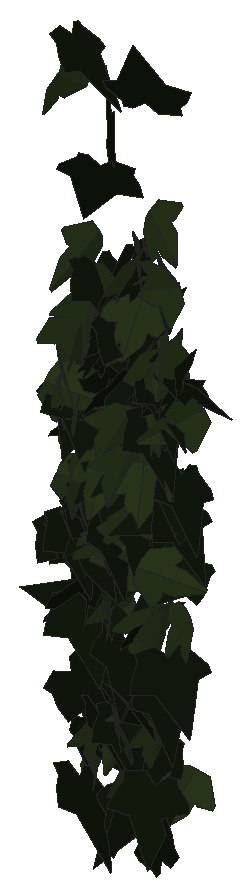
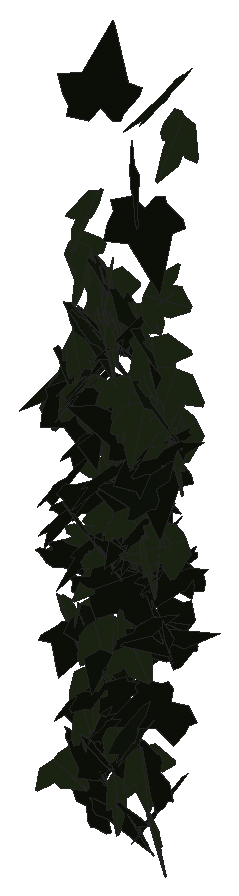
# SketchUp Ruby script. Lengths in inches.
U = 1.inch
M = Sketchup.active_model
def pt(a) = Geom::Point3d.new(a.map { |v| v * U })
def face(e, loops, mat)
  f = e.add_face(loops[0].map { |a| pt(a) })
  loops[1..].each { |l| e.add_face(l.map { |a| pt(a) }).erase! }
  f.material = f.back_material = mat if mat
  f
end
# faces: each face lists its corners as indices into pts; further lists are holes
def faces(e, pts, list, mat = nil) = list.each { |f| face(e, (f[0].is_a?(Array) ? f : [f]).map { |l| l.map { |i| pts[i] } }, mat) }
# xy, xz, yz: faces in a plane at the given z, y or x. An outline is a flat list of corners, or four numbers for a rectangle; further outlines are holes
def ring(l) = l.size == 4 ? [[l[0], l[1]], [l[2], l[1]], [l[2], l[3]], [l[0], l[3]]] : l.each_slice(2).to_a
def flat(e, list, mat, &to3) = list.each { |f| face(e, (f[0].is_a?(Array) ? f : [f]).map { |l| ring(l).map { |u, v| to3.(u, v) } }, mat) }
def xy(e, z, list, mat = nil) = flat(e, list, mat) { |x, y| [x, y, z] }
def xz(e, y, list, mat = nil) = flat(e, list, mat) { |x, z| [x, y, z] }
def yz(e, x, list, mat = nil) = flat(e, list, mat) { |y, z| [x, y, z] }
def lines(e, pts, list) = list.each { |a, b| e.add_line(pt(pts[a]), pt(pts[b])) }
# prism: a flat outline (further loops are holes) pulled along v
def prism(e, loops, v, mat = nil)
  f = face(e, loops, mat); d = Geom::Vector3d.new(v.map { |x| x * U })
  f.pushpull(f.normal.samedirection?(d) ? d.length : -d.length)
end
def box(e, o, s, mat = nil) = prism(e, [[o, [o[0] + s[0], o[1], o[2]], [o[0] + s[0], o[1] + s[1], o[2]], [o[0], o[1] + s[1], o[2]]]], [0, 0, s[2]], mat)
def at(x, y, z, deg = 0) = Geom::Transformation.translation(pt([x, y, z])) * Geom::Transformation.rotation(ORIGIN, Z_AXIS, deg.degrees)
def axes(o, x, y, z) = Geom::Transformation.new([*x, 0, *y, 0, *z, 0, *pt(o).to_a, 1])
def part(name) = M.definitions.add(name)
# library, detail: a bought-in or finely detailed component or shape, given as its bounding box
def library(name, o, s) = part(name).tap { |d| box(d.entities, o, s) }
def detail(e, o, s) = box(e.add_group.entities, o, s)
def put(e, d, t, mat = nil) = e.add_instance(d, t).tap { |i| i.material = mat if mat }
def group(e, t, mat = nil) = e.add_group.tap { |g| g.transformation = t; g.material = mat if mat }.entities
root = M.entities
M.materials.add("efeu1").color = [18, 25, 13]
M.materials.add("efeu2").color = [43, 57, 29]
c1 = part("ivyleaf_9")
p = [[1.54,2.16,1.25],[1.36,2.04,1.19],[-0.21,0.99,0.68],[-0.71,1.11,0.82],[-0.85,0.86,0.67],[-0.8,0.17,0.21],
  [-0.9,-0.01,0.1],[-0.67,-0.16,-0.02],[-0.08,-0.08,-0.05],[-0.03,-0.6,-0.4],[0.65,-0.88,-0.66],[0.83,-0.6,-0.49],
  [1.29,-0.42,-0.43],[1.8125,-0.07,-0.26],[1.21,0.44,0.15]]
faces(c1.entities,p,[[0,1,2,3,4,5,6,7,8,9,10,11,12,13,14]],"efeu1")
c2 = part("ivyleaf_10")
p = [[0,0.5,-0.03],[-0.0625,2.02,-0.43],[-0.19,2.01,-0.46],[-0.54,1.05,-0.29],[-0.52,0.625,-0.18],[-0.83,0.76,-0.28],
  [-1.16,0.64,-0.33],[-1.15,0.33,-0.24],[-0.77,-0.39,0.02],[-0.3,-0.51,0.16],[0.04,-0.48,0.23],[-0.02,2.01,-0.4375],
  [-0.06,2.01,-0.43],[0.04,-0.49,0.23],[0.67,-0.49,0.14],[1.38,0.36,-0.2],[1.375,0.51,-0.24],[0.81,0.65,-0.19],
  [0.62,0.59,-0.15],[0.6,1.09,-0.28],[0.5,1.23,-0.31]]
faces(c2.entities,p,[[0,1,2,3,4,5,6,7,8,9,10],[11,12,0,13,14,15,16,17,18,19,20]],"efeu2")
put(root,c1,axes([551.22,132.15,207.84],[-0.35573,-0.80751,-0.25845],[0.08409,0.24529,-0.88214],[0.84368,-0.36493,-0.02105]))
put(root,c1,axes([550.91,132.11,233.63],[0.90126,0.01452,0.45871],[-0.45894,0.03227,0.90069],[-0.00171,-1.01077,0.03534]))
put(root,c2,axes([550.11,132.13,219.92],[-0.28181,-0.82946,0.30019],[-0.04556,-0.30103,-0.87455],[0.88093,-0.28091,0.0508]))
put(root,c2,axes([548.48,131.66,224.34],[0.38067,-0.79091,-0.40343],[-0.03419,0.42556,-0.86657],[0.88721,0.35576,0.1397]))
put(root,c2,axes([548.13,132.57,227.09],[-0.01841,-0.48837,0.86162],[0.11843,-0.85667,-0.48304],[0.9833,0.09403,0.07431]))
put(root,c2,axes([552.15,131.71,227.17],[0.42257,-0.0171,-0.82934],[-0.77192,0.33266,-0.40018],[0.3037,0.86931,0.13682]))
put(root,c1,axes([550.09,132.42,210.54],[0.18303,-0.59002,0.61117],[0.43229,-0.4735,-0.58658],[0.73128,0.42758,0.19378]))
put(root,c1,axes([548.01,132,234.99],[0.57668,-0.76119,-0.19476],[0.0176,0.25404,-0.94077],[0.78551,0.55313,0.16406]))
put(root,c2,axes([551.29,132.24,224.59],[0.75505,-0.33149,0.41588],[0.38532,-0.15679,-0.82455],[0.36656,0.84763,0.01012]))
put(root,c2,axes([548.4375,131.46,218.76],[0.18882,-0.41507,-0.79085],[0.06201,0.81247,-0.41162],[0.891,0.03142,0.19624]))
put(root,c1,axes([548.39,132.22,213.72],[-0.36618,-0.70373,-0.51272],[0.30488,0.41737,-0.79061],[0.81558,-0.47199,0.06534]))
put(root,c1,axes([549.17,132.41,216.79],[0.29275,-0.84359,0.13417],[0.04835,-0.12524,-0.89293],[0.85282,0.29668,0.00457]))
put(root,c2,axes([549.77,132.39,221.19],[-0.33472,-0.75707,0.42071],[-0.13553,-0.39969,-0.82709],[0.85545,-0.35956,0.03358]))
put(root,c1,axes([547.98,132.35,206.93],[0.49014,-0.98605,0.00574],[0.0103,-0.00129,-1.10111],[0.98601,0.49017,0.00865]))
put(root,c2,axes([550.47,132.19,225.58],[0.907,0.16,-0.15561],[-0.15258,-0.03079,-0.92099],[-0.1629,0.91973,-0.00376]))
put(root,c2,axes([549.05,132.24,219.27],[0.51065,0.72235,-0.26572],[-0.15716,-0.2143,-0.88461],[-0.75346,0.53427,0.00443]))
put(root,c2,axes([547.5,131.82,221.87],[-0.28578,-0.27746,-0.85204],[0.79855,0.32687,-0.37428],[0.40653,-0.83713,0.13625]))
put(root,c2,axes([551.46,132.1,224.16],[-0.35992,-0.83798,-0.1657],[0.13284,0.12272,-0.90912],[0.84381,-0.37675,0.07244]))
put(root,c2,axes([547.76,132.18,221.22],[0.67839,-0.57257,-0.16024],[-0.0978,0.13233,-0.88693],[0.58647,0.68438,0.03744]))
put(root,c2,axes([551.61,131.79,229.39],[-0.14847,0.8548,0.34443],[-0.05869,0.3394,-0.8676],[-0.91971,-0.15965,-0.00024]))
put(root,c2,axes([549.24,131.97,216.77],[-0.57712,-0.58599,-0.40281],[0.32941,0.23944,-0.82029],[0.63019,-0.66182,0.05989]))
put(root,c2,axes([550.58,132.25,219.28],[0.90123,0.14198,0.03758],[0.03716,0.00565,-0.91235],[-0.14209,0.902,-0.0002]))
put(root,c1,axes([551.58,131.97,205.51],[0.09333,-0.12126,0.90251],[-0.5925,0.68085,0.15275],[-0.6915,-0.59973,-0.00907]))
put(root,c1,axes([547.58,132.375,216.5],[0.19749,-0.84521,-0.21545],[-0.04014,0.21186,-0.86793],[0.87132,0.20133,0.00885]))
put(root,c1,axes([549.59,132.71,212.36],[0.00636,-0.90084,0.18203],[0.00852,-0.18197,-0.90083],[0.91901,0.00792,0.00709]))
put(root,c2,axes([547.41,132.13,222.79],[-0.42101,0.8124,-0.10164],[0.06596,-0.08027,-0.91476],[-0.81607,-0.42561,-0.0215]))
put(root,c1,axes([547.99,132.21,216.61],[-0.29699,-0.36346,-0.83752],[0.60473,0.5815,-0.46679],[0.68398,-0.67194,0.04905]))
put(root,c1,axes([548.07,132.26,217.34],[0.52925,-0.69391,-0.2124],[-0.0639,0.2173,-0.86916],[0.72287,0.52725,0.07868]))
put(root,c1,axes([549.09,132.73,217.89],[-0.76802,-0.46735,0.06719],[-0.05694,-0.03568,-0.89903],[0.4687,-0.77013,0.00088]))
put(root,c1,axes([549.22,132.76,219.47],[-0.7939,-0.41525,0.13081],[-0.10467,-0.08203,-0.89562],[0.4226,-0.80041,0.02392]))
put(root,c2,axes([547.68,131.75,233.625],[-0.09897,-0.6513,-0.78315],[0.06875,0.78077,-0.65801],[1.01626,-0.11625,-0.03175]))
put(root,c2,axes([549.625,132.7,209.44],[-0.17898,-0.74572,0.42865],[0.04333,-0.4451,-0.75623],[0.85905,-0.13292,0.12746]))
put(root,c1,axes([547.75,132.66,221.375],[-0.06751,-0.91605,-0.14778],[0.03265,0.14574,-0.91828],[0.92732,-0.07183,0.02157]))
put(root,c2,axes([551.2,132.1,216.05],[-0.25726,-0.1989,-0.85564],[0.84426,0.19035,-0.29809],[0.24271,-0.87296,0.12996]))
put(root,c2,axes([549.84,132.04,209.65],[-0.64053,0.30898,0.61131],[-0.5702,0.22322,-0.71027],[-0.37953,-0.85682,0.03541]))
put(root,c1,axes([548.67,132.63,209.625],[0.42702,-0.75705,0.14353],[0.08712,-0.11561,-0.86897],[0.7656,0.43541,0.01883]))
put(root,c1,axes([550.73,132.39,227.3],[-0.7771,0.50984,-0.07614],[0.03786,-0.08091,-0.92824],[-0.5141,-0.77662,0.04673]))
put(root,c1,axes([551.24,132.15,224.74],[-0.50884,0.50559,0.58216],[-0.51617,0.29481,-0.70719],[-0.57281,-0.71479,0.12011]))
put(root,c1,axes([547.59,131.67,213.64],[0.41514,0.27726,0.73871],[0.45135,0.60122,-0.4793],[-0.64719,0.59714,0.13958]))
put(root,c2,axes([549.35,132.33,219.33],[-0.82082,-0.25882,0.28159],[-0.27605,-0.06056,-0.86033],[0.26473,-0.86566,-0.024]))
put(root,c2,axes([552.26,132.78,221.9],[0.16986,0.36987,-0.83067],[-0.68051,-0.50876,-0.36569],[-0.60309,0.67825,0.17868]))
put(root,c2,axes([547.61,132.4,221.77],[0.12268,0.89001,-0.16681],[-0.11958,-0.15093,-0.89326],[-0.89758,0.14176,0.0962]))
put(root,c2,axes([550.03,132.46,226.87],[0.09124,-0.94807,-0.05139],[0.00309,0.05192,-0.95242],[0.94946,0.09094,0.00804]))
put(root,c1,axes([551.61,132.47,212.64],[-0.24607,-0.68822,-0.55777],[0.21299,0.51595,-0.73058],[0.85988,-0.32475,0.02134]))
put(root,c1,axes([549.63,132.3,224.82],[0.39168,-0.71642,-0.47501],[-0.04522,0.50411,-0.79759],[0.8584,0.35345,0.17473]))
put(root,c1,axes([549.57,131.92,222.49],[-0.03994,0.92139,0.12156],[0.01586,0.12233,-0.92202],[-0.92924,-0.03751,-0.02097]))
put(root,c1,axes([548.5,132.58,226.27],[0.26992,-0.87248,-0.2569],[-0.0193,0.26242,-0.9115],[0.90931,0.26455,0.05691]))
put(root,c1,axes([547.86,132.16,210.95],[0.07653,-0.1347,-0.92948],[0.552,0.76094,-0.06482],[0.75985,-0.53922,0.14071]))
put(root,c1,axes([548.33,132.79,213.41],[-0.37452,0.04394,0.80373],[-0.79665,-0.14707,-0.36318],[0.11517,-0.87443,0.10147]))
put(root,c2,axes([547.59,132.39,223.89],[-0.7636,-0.49705,-0.23383],[0.24973,0.04252,-0.90589],[0.48926,-0.79746,0.09744]))
put(root,c2,axes([548.17,132.6,224.97],[-0.40435,-0.84929,0.10834],[0.01381,-0.12627,-0.9383],[0.85606,-0.39911,0.06631]))
put(root,c1,axes([549.6,132.65,209.85],[0.03999,-0.83472,-0.27833],[-0.02422,0.27746,-0.83561],[0.87957,0.0456,-0.01036]))
put(root,c2,axes([549.1875,132.45,225.95],[-0.84437,0.10526,0.34407],[-0.35694,-0.13427,-0.83486],[-0.04541,-0.90184,0.16446]))
put(root,c1,axes([549.37,132.17,205.44],[-0.59316,0.71334,0.38975],[0.24095,-0.30651,0.92768],[0.77634,0.64016,0.00987]))
put(root,c1,axes([548.77,132.35,230.22],[0.47536,0.57918,-0.65463],[-0.43627,-0.48851,-0.749],[-0.75741,0.64489,0.02056]))
put(root,c1,axes([547.35,132.49,216.35],[-0.0258,-0.68991,-0.5944],[0.21109,0.57391,-0.6753],[0.88585,-0.15685,0.1436]))
put(root,c2,axes([550.79,132.56,221.28],[0.77413,-0.46189,-0.12351],[-0.07795,0.10997,-0.89983],[0.47172,0.77616,0.054]))
put(root,c2,axes([550.39,132.93,215.76],[-0.09467,0.25205,0.89208],[-0.613,-0.6897,0.12982],[0.69539,-0.57366,0.23588]))
put(root,c1,axes([549.23,132.06,223.6],[-0.06463,0.12449,0.9838],[-0.4568,0.87132,-0.14026],[-0.88017,-0.46135,0.00056]))
put(root,c2,axes([549.84,133.09,226.62],[-0.10047,0.01502,1.02934],[0.82774,-0.61371,0.08975],[0.61205,0.83246,0.0476]))
put(root,c2,axes([550.1,132.3,217.66],[-0.47699,-0.58391,-0.49781],[0.40538,0.3059,-0.74724],[0.65148,-0.61786,0.10049]))
put(root,c2,axes([548.91,133.15,213.49],[0.06646,-0.47004,-0.76344],[0.08508,-0.75877,0.47458],[-0.89249,-0.10733,-0.01161]))
put(root,c2,axes([551.4,132.4,227.37],[-0.72166,0.5894,0.02654],[-0.02492,0.01145,-0.93174],[-0.58947,-0.72205,0.00689]))
put(root,c1,axes([552.03,132.49,223.29],[-0.68646,0.64382,-0.03567],[0.02218,-0.02849,-0.94112],[-0.64443,-0.6868,0.0056]))
put(root,c1,axes([547.51,133.125,221.23],[-0.30488,-0.86682,0.09621],[0.01011,-0.10542,-0.91781],[0.87208,-0.30182,0.04428]))
put(root,c2,axes([548.26,132.17,217.3125],[-0.49613,0.42686,0.67185],[-0.5058,0.44222,-0.65447],[-0.61461,-0.7085,-0.00372]))
put(root,c1,axes([550.86,132.84,223.02],[0.34504,-0.85898,-0.14585],[-0.01381,0.15146,-0.92468],[0.87116,0.34261,0.04311]))
put(root,c1,axes([551.49,133.21,218.19],[-0.61275,-0.38127,0.52399],[-0.45795,-0.25546,-0.7214],[0.4585,-0.7647,-0.02026]))
put(root,c1,axes([549.82,133,206.48],[-0.85192,-0.22979,-0.15515],[0.15433,0.02347,-0.88219],[0.23034,-0.86561,0.01726]))
put(root,c1,axes([548.68,132.625,223.58],[-0.69134,0.6085,-0.06336],[0.03831,-0.05235,-0.92089],[-0.61059,-0.69226,0.01395]))
put(root,c1,axes([549.49,132.49,226.41],[-0.56666,0.72273,0.07352],[-0.03163,0.06861,-0.91823],[-0.72577,-0.56728,-0.01738]))
put(root,c1,axes([548.41,132.17,213.87],[-0.09595,0.22694,0.95168],[-0.40508,0.86122,-0.24621],[-0.89057,-0.41618,0.00945]))
put(root,c1,axes([550.88,133.07,222.62],[0.17445,-0.91011,-0.0057],[-0.00408,0.00502,-0.92668],[0.91012,0.17447,-0.00307]))
put(root,c1,axes([548.39,133.12,217.39],[0.0718,-0.89474,-0.00496],[-0.00532,0.00455,-0.8976],[0.89474,0.07183,-0.00494]))
put(root,c1,axes([548.19,132.44,220.46],[0.27759,0.82426,-0.3033],[-0.2048,-0.24858,-0.86297],[-0.85408,0.3275,0.10836]))
put(root,c1,axes([550.54,133,221.04],[0.13671,-0.88224,-0.24414],[-0.02318,0.24343,-0.89266],[0.91511,0.13797,0.01386]))
put(root,c2,axes([549.09,132.91,213.89],[-0.02825,-0.92668,0.01137],[0.00025,-0.01139,-0.92711],[0.92675,-0.02825,0.0006]))
put(root,c2,axes([551.33,132.89,224.13],[0.12467,-0.92554,-0.0414],[0.00184,0.04202,-0.93387],[0.92646,0.12446,0.00743]))
put(root,c1,axes([548.65,132.3,218.87],[0.74579,0.6399,0.01935],[0.01481,0.01246,-0.98269],[-0.64002,0.74594,-0.00019]))
put(root,c1,axes([549.8,133.06,208.1875],[0.76736,0.18996,0.45125],[-0.43974,-0.10147,0.7905],[0.21527,-0.8844,0.00622]))
put(root,c2,axes([549.76,133,225.45],[-0.71601,0.46987,-0.34019],[0.13636,-0.38894,-0.8242],[-0.56384,-0.69075,0.23268]))
put(root,c2,axes([550.84,132.94,213.79],[0.00674,-0.87329,-0.03008],[0.05601,0.03045,-0.87151],[0.87201,0.0048,0.05621]))
put(root,c2,axes([550.8,132.98,209.71],[-0.08908,-0.87599,0.02683],[0.00021,-0.02699,-0.88051],[0.8764,-0.08903,0.00294]))
put(root,c1,axes([551.04,132.88,225.27],[-0.75045,0.53768,0.05749],[-0.09593,-0.0356,-0.91929],[-0.53217,-0.7518,0.08464]))
put(root,c1,axes([548.73,132.65,221.58],[0.36348,-0.13118,0.84205],[0.85142,0.09526,-0.35269],[-0.03664,0.91219,0.15792]))
put(root,c1,axes([551.29,132.71,225.29],[-0.57312,0.7143,0.15475],[-0.11369,0.10713,-0.91555],[-0.72198,-0.5839,0.02133]))
put(root,c2,axes([548.32,133.01,208.85],[-0.19007,-0.88496,-0.00511],[0.00033,0.00516,-0.90514],[0.88497,-0.19007,-0.00076]))
put(root,c1,axes([551.9,133.34,216.0625],[-0.8442,-0.25635,0.1619],[-0.15489,-0.04711,-0.88227],[0.26065,-0.85829,0.00007]))
put(root,c2,axes([550.73,132.58,226.71],[-0.50789,0.2847,0.735],[-0.66586,0.31293,-0.58133],[-0.4218,-0.83681,0.03267]))
put(root,c1,axes([547.56,133.12,208.6875],[0.11981,-0.13014,-0.86664],[0.83704,0.27606,0.07426],[0.25956,-0.83019,0.16055]))
put(root,c1,axes([549.54,133.16,215.66],[0.18819,0.19068,-0.91303],[-0.60694,-0.68222,-0.26758],[-0.70824,0.6353,-0.0133]))
put(root,c1,axes([549.83,133.5,211.26],[-0.47179,-0.85626,-0.04424],[0.02976,0.03411,-0.97759],[0.85689,-0.47263,0.0096]))
put(root,c1,axes([551.49,133.32,219.11],[0.19526,-0.89312,-0.04346],[0.00259,0.04504,-0.91414],[0.89418,0.1949,0.01214]))
put(root,c1,axes([549.16,132.5,230.87],[0.0479,-0.18226,1.01157],[-0.17514,0.99641,0.18782],[-1.01283,-0.18092,0.01536]))
put(root,c1,axes([550.87,133.27,208.86],[-0.79733,-0.09498,-0.35517],[0.35142,0.0523,-0.80291],[0.10801,-0.87129,-0.00948]))
put(root,c2,axes([550.8,133.26,222.74],[-0.50976,-0.71089,0.27947],[-0.07556,-0.28741,-0.86892],[0.76011,-0.50533,0.10105]))
put(root,c1,axes([551.31,132.71,223.23],[0.84274,-0.32966,-0.17543],[-0.02954,0.37283,-0.84249],[0.37226,0.77587,0.3303]))
put(root,c2,axes([548.18,133.18,218.36],[0.89411,-0.0799,0.05219],[0.05107,-0.01482,-0.89762],[0.08062,0.89551,-0.01019]))
put(root,c2,axes([550.03,133.0625,225.59],[0.6951,-0.57535,-0.20468],[-0.10839,0.18896,-0.89924],[0.60098,0.69954,0.07456]))
put(root,c2,axes([551.72,133.04,213.8],[0.67662,-0.45975,-0.34866],[-0.27497,0.21546,-0.81774],[0.50726,0.73003,0.02178]))
put(root,c2,axes([548.48,133.18,218.45],[-0.70384,-0.59327,0.01785],[0.12025,-0.16965,-0.8969],[0.58123,-0.68333,0.20718]))
put(root,c1,axes([550.3,132.86,216.92],[0.36196,-0.58741,-0.57975],[-0.12324,0.58749,-0.67219],[0.81607,0.34926,0.15563]))
put(root,c1,axes([550.02,133.11,222.66],[-0.34015,-0.58215,-0.63417],[0.29242,0.5632,-0.67384],[0.80967,-0.44797,-0.02306]))
put(root,c1,axes([547.74,133.15,219.94],[0.64276,-0.50011,0.43505],[0.4552,-0.10748,-0.79609],[0.48184,0.76867,0.17173]))
put(root,c2,axes([550.08,133.33,213.4],[-0.25508,-0.85325,0.20204],[0.02646,-0.21781,-0.88644],[0.87644,-0.24175,0.08557]))
put(root,c2,axes([551.7,133.42,207.73],[0.42559,0.58591,-0.52228],[-0.29945,-0.42798,-0.72413],[-0.72554,0.52032,-0.0075]))
put(root,c1,axes([550.61,133.43,210.9],[0.10056,-0.88852,-0.10206],[-0.02612,0.09974,-0.89407],[0.89398,0.10286,-0.01465]))
put(root,c1,axes([549.61,133.45,217.22],[-0.8769,-0.14765,-0.1341],[0.13097,0.02979,-0.88921],[0.15043,-0.8866,-0.00754]))
put(root,c1,axes([551.3125,133.28,217.85],[0.23423,-0.82469,-0.26147],[0.01342,0.27431,-0.85318],[0.86505,0.21905,0.08403]))
put(root,c2,axes([549.4,133.12,207.55],[0.11296,-0.82793,-0.16248],[0.0212,0.16666,-0.8345],[0.84345,0.10669,0.04274]))
put(root,c1,axes([551.15,133.07,222.43],[0.21932,0.72452,-0.53264],[-0.15657,-0.50911,-0.75699],[-0.88551,0.26946,0.00193]))
put(root,c2,axes([550.03,132.79,216.14],[-0.2598,-0.57015,-0.64392],[0.40833,0.51024,-0.61654],[0.75695,-0.47093,0.11158]))
put(root,c2,axes([548.51,133.32,213.45],[0.28807,0.78096,-0.33312],[-0.24446,-0.26058,-0.82231],[-0.81308,0.35503,0.12921]))
put(root,c2,axes([548.875,133.1,223.41],[-0.80072,-0.43922,-0.06667],[0.05335,0.04135,-0.91321],[0.44104,-0.80242,-0.01057]))
put(root,c2,axes([548.23,133.16,222.62],[-0.62155,-0.64557,-0.1632],[0.17885,0.05319,-0.89158],[0.64141,-0.64042,0.09046]))
put(root,c1,axes([547.87,133.16,218.55],[0.26901,-0.71925,-0.46522],[-0.16517,0.43492,-0.7679],[0.84052,0.31566,-0.00201]))
put(root,c2,axes([547.9,133.3,217.6],[0.28867,-0.86911,-0.03695],[0.01691,0.04453,-0.9153],[0.86973,0.2876,0.03006]))
put(root,c2,axes([550.7,133.09,211.22],[-0.77032,0.16838,0.33576],[-0.33773,0.02478,-0.78728],[-0.16438,-0.83995,0.04408]))
put(root,c1,axes([549.45,133.16,220.15],[0.37087,-0.72019,-0.42667],[0.00962,0.4703,-0.78548],[0.83704,0.31369,0.19807]))
put(root,c2,axes([547.12,132.91,217.85],[-0.26711,-0.16322,-0.85574],[0.78921,0.33366,-0.30999],[0.36888,-0.83205,0.04356]))
put(root,c1,axes([547.99,133.83,214.41],[-0.34174,-0.79021,0.20626],[-0.04167,-0.20643,-0.85989],[0.81562,-0.34164,0.04249]))
put(root,c1,axes([549.95,133.76,215.91],[-0.64814,-0.60345,0.08908],[-0.06607,-0.05977,-0.88557],[0.6064,-0.65149,-0.00127]))
put(root,c1,axes([548.36,133.4,210.28],[0.59044,-0.62037,0.05149],[0.03476,-0.03799,-0.85643],[0.62153,0.59146,-0.00101]))
put(root,c1,axes([550.41,132.81,213.49],[0.06094,0.86553,0.07416],[0.02908,0.07227,-0.86735],[-0.86822,0.06318,-0.02385]))
put(root,c1,axes([551.15,133.16,217.53],[-0.71954,0.52157,0.2293],[-0.17983,0.14259,-0.88864],[-0.54062,-0.74161,-0.00959]))
put(root,c2,axes([547.6875,133.24,206.59],[0.51876,-0.6228,-0.29877],[-0.19736,0.22443,-0.81051],[0.66196,0.55498,-0.00751]))
